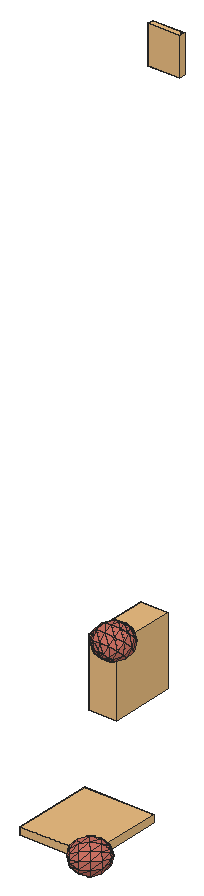
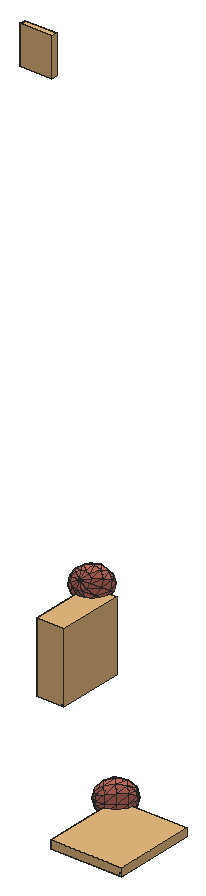
# SketchUp Ruby script. Lengths in inches.
U = 1.inch
M = Sketchup.active_model
def pt(a) = Geom::Point3d.new(a.map { |v| v * U })
def face(e, loops, mat)
  f = e.add_face(loops[0].map { |a| pt(a) })
  loops[1..].each { |l| e.add_face(l.map { |a| pt(a) }).erase! }
  f.material = f.back_material = mat if mat
  f
end
# faces: each face lists its corners as indices into pts; further lists are holes
def faces(e, pts, list, mat = nil) = list.each { |f| face(e, (f[0].is_a?(Array) ? f : [f]).map { |l| l.map { |i| pts[i] } }, mat) }
# xy, xz, yz: faces in a plane at the given z, y or x. An outline is a flat list of corners, or four numbers for a rectangle; further outlines are holes
def ring(l) = l.size == 4 ? [[l[0], l[1]], [l[2], l[1]], [l[2], l[3]], [l[0], l[3]]] : l.each_slice(2).to_a
def flat(e, list, mat, &to3) = list.each { |f| face(e, (f[0].is_a?(Array) ? f : [f]).map { |l| ring(l).map { |u, v| to3.(u, v) } }, mat) }
def xy(e, z, list, mat = nil) = flat(e, list, mat) { |x, y| [x, y, z] }
def xz(e, y, list, mat = nil) = flat(e, list, mat) { |x, z| [x, y, z] }
def yz(e, x, list, mat = nil) = flat(e, list, mat) { |y, z| [x, y, z] }
def lines(e, pts, list) = list.each { |a, b| e.add_line(pt(pts[a]), pt(pts[b])) }
# prism: a flat outline (further loops are holes) pulled along v
def prism(e, loops, v, mat = nil)
  f = face(e, loops, mat); d = Geom::Vector3d.new(v.map { |x| x * U })
  f.pushpull(f.normal.samedirection?(d) ? d.length : -d.length)
end
def box(e, o, s, mat = nil) = prism(e, [[o, [o[0] + s[0], o[1], o[2]], [o[0] + s[0], o[1] + s[1], o[2]], [o[0], o[1] + s[1], o[2]]]], [0, 0, s[2]], mat)
def at(x, y, z, deg = 0) = Geom::Transformation.translation(pt([x, y, z])) * Geom::Transformation.rotation(ORIGIN, Z_AXIS, deg.degrees)
def axes(o, x, y, z) = Geom::Transformation.new([*x, 0, *y, 0, *z, 0, *pt(o).to_a, 1])
def part(name) = M.definitions.add(name)
# library, detail: a bought-in or finely detailed component or shape, given as its bounding box
def library(name, o, s) = part(name).tap { |d| box(d.entities, o, s) }
def detail(e, o, s) = box(e.add_group.entities, o, s)
def put(e, d, t, mat = nil) = e.add_instance(d, t).tap { |i| i.material = mat if mat }
def group(e, t, mat = nil) = e.add_group.tap { |g| g.transformation = t; g.material = mat if mat }.entities
root = M.entities
M.materials.add("green").color = [174, 139, 102]
M.materials.add("vio").color = [206, 114, 100]
c1 = part("3DGeom~190_Defintion")
p = [[103.5625,-60.76,-498.22],[-159.65,90.28,-476.73],[101.5,52.12,-500],[335.44,0,-389.29],[150.07,151.03,-458.14],[-75.51,261.6,-404.23],
  [155.72,-157.36,-453.28],[-156.07,-105.24,-473.65],[-378.01,104.24,-325.73],[-280.86,302.07,-242.01],[-280.86,302.07,-242.01],[-65.73,-272.55,-395.81],
  [-373.88,-121.52,-322.17],[236.28,209.48,-383.86],[73.81,362.83,-275.57],[73.81,362.83,-275.57],[243.99,-211.79,-377.22],[-75.51,261.6,-404.23],
  [-280.86,302.07,-242.01],[-108.44,418.95,-93.44],[-75.51,261.6,-404.23],[73.81,362.83,-275.57],[87.16,-366.83,-264.07],[-269.57,-314.71,-232.28],
  [-65.73,-272.55,-395.81],[87.16,-366.83,-264.07],[-269.57,-314.71,-232.28],[344.72,-209.48,-290.42],[430.93,-151.03,-216.13],[344.72,-209.48,-290.42],
  [335.44,0,-389.29],[479.51,-52.12,-174.27],[335.44,0,-389.29],[477.44,60.76,-176.05],[335.44,0,-389.29],[337.02,211.79,-297.06],
  [425.29,157.36,-221],[335.44,0,-389.29],[337.02,211.79,-297.06],[335.44,0,-389.29],[236.28,209.48,-383.86],[248.29,366.83,-125.23],
  [236.28,209.48,-383.86],[248.29,366.83,-125.23],[337.02,211.79,-297.06],[344.72,-209.48,-290.42],[87.16,-366.83,-264.07],[243.99,-211.79,-377.22],
  [-373.88,-121.52,-322.17],[-495.09,90.28,-87.4375],[-378.01,104.24,-325.73],[-378.01,104.24,-325.73],[-410.95,261.6,-14.9375],[-378.01,104.24,-325.73],
  [-410.95,261.6,-14.9375],[-280.86,302.07,-242.01],[-269.57,-314.71,-232.28],[-491.51,-105.24,-84.36],[-373.88,-121.52,-322.17],[-373.88,-121.52,-322.17],
  [401.18,272.55,6.52],[248.29,366.83,-125.23],[344.72,-209.48,-290.42],[261.64,-362.83,-113.72],[87.16,-366.83,-264.07],[261.64,-362.83,-113.72],
  [344.72,-209.48,-290.42],[93.03,423.58,80.16],[248.29,366.83,-125.23],[87.16,-366.83,-264.07],[-93.03,-423.58,-80.16],[-269.57,-314.71,-232.28],
  [87.16,-366.83,-264.07],[-410.95,261.6,-14.9375],[-261.64,362.83,113.72],[-401.18,-272.55,-6.52],[-269.57,-314.71,-232.28],[-269.57,-314.71,-232.28],
  [-401.18,-272.55,-6.52],[491.51,105.23,84.36],[410.95,-261.6,14.9375],[261.64,-362.83,-113.72],[495.09,-90.28,87.44],[248.29,366.83,-125.23],
  [269.57,314.71,232.28],[401.18,272.55,6.52],[248.29,366.83,-125.23],[269.57,314.71,232.28],[108.44,-418.95,93.44],[410.95,-261.6,14.9375],
  [-87.16,366.83,264.07],[-479.51,52.12,174.27],[-430.93,151.03,216.13],[-410.95,261.6,-14.9375],[-477.44,-60.76,176.05],[-248.29,-366.83,125.23],
  [-401.18,-272.55,-6.52],[-410.95,261.6,-14.9375],[-344.72,209.48,290.42],[-410.95,261.6,-14.9375],[-344.72,209.48,290.42],[-261.64,362.83,113.72],
  [-248.29,-366.83,125.23],[-425.29,-157.36,221],[373.88,121.52,322.17],[269.57,314.71,232.28],[410.95,-261.6,14.9375],[280.86,-302.07,242.01],
  [280.86,-302.07,242.01],[65.73,272.55,395.81],[65.73,272.55,395.81],[269.57,314.71,232.28],[378.01,-104.24,325.73],[280.86,-302.07,242.01],
  [-73.81,-362.83,275.57],[-344.72,209.48,290.42],[-243.99,211.79,377.22],[-243.99,211.79,377.22],[-248.29,-366.83,125.23],[-337.02,-211.79,297.06],
  [-337.02,-211.79,297.06],[-335.44,0,389.29],[-344.72,209.48,290.42],[269.57,314.71,232.28],[65.73,272.55,395.81],[156.07,105.24,473.65],
  [269.57,314.71,232.28],[373.88,121.52,322.17],[75.51,-261.6,404.23],[378.01,-104.24,325.73],[75.51,-261.6,404.23],[280.86,-302.07,242.01],
  [-87.16,366.83,264.07],[-243.99,211.79,377.22],[-155.72,157.36,453.28],[-87.16,366.83,264.07],[-236.28,-209.48,383.86],[-337.02,-211.79,297.06],
  [75.51,-261.6,404.23],[-236.28,-209.48,383.86],[-73.81,-362.83,275.57],[-344.72,209.48,290.42],[-335.44,0,389.29],[-337.02,-211.79,297.06],
  [-236.28,-209.48,383.86],[-335.44,0,389.29],[373.88,121.52,322.17],[159.65,-90.28,476.73],[378.01,-104.24,325.73],[373.88,121.52,322.17],
  [378.01,-104.24,325.73],[75.51,-261.6,404.23],[-335.44,0,389.29],[75.51,-261.6,404.23],[-150.07,-151.03,458.14],[-236.28,-209.48,383.86],
  [-236.28,-209.48,383.86],[-335.44,0,389.29],[-101.5,-52.12,500],[-335.44,0,389.29],[-103.5625,60.76,498.22],[-335.44,0,389.29],
  [-335.44,0,389.29],[75.51,-261.6,404.23]]
faces(c1.entities,p,[[0,1,2],[0,2,3],[2,4,3],[2,1,5],[2,5,4],[6,7,0],[6,0,3],[0,7,1],
  [7,8,1],[1,8,9],[1,10,5],[11,12,7],[6,11,7],[7,12,8],[4,13,3],[4,5,14],
  [4,15,13],[16,11,6],[16,6,3],[17,18,19],[20,19,21],[22,23,24],[16,25,11],[11,26,12],
  [27,16,3],[28,29,30],[31,28,32],[33,31,34],[13,35,3],[36,33,37],[38,36,39],[40,21,41],
  [42,43,44],[45,46,47],[48,49,50],[51,49,52],[53,54,55],[56,57,58],[59,57,49],[38,60,36],
  [38,61,60],[62,63,64],[28,65,66],[21,19,67],[21,67,68],[69,70,71],[63,70,72],[18,73,74],
  [18,74,19],[70,75,76],[77,78,57],[36,79,33],[36,60,79],[28,80,81],[31,80,28],[33,79,82],
  [33,82,31],[31,82,80],[83,84,85],[86,67,87],[63,88,70],[89,88,63],[19,74,90],[19,90,67],
  [57,91,49],[49,91,92],[49,92,93],[78,94,57],[57,94,91],[70,95,96],[88,95,70],[97,92,98],
  [99,100,101],[102,103,78],[78,103,94],[60,104,79],[60,105,104],[106,107,88],[82,108,80],[67,90,109],
  [67,110,111],[79,104,112],[79,112,82],[82,112,113],[88,114,95],[107,114,88],[74,115,116],[74,117,90],
  [118,119,103],[114,120,95],[91,94,121],[92,91,121],[94,103,121],[122,92,121],[103,119,121],[123,124,125],
  [126,125,127],[107,128,114],[129,130,131],[132,133,134],[135,134,124],[114,136,137],[138,139,140],[133,141,142],
  [143,144,145],[146,147,148],[149,125,147],[150,147,151],[134,133,152],[153,154,155],[156,154,157],[154,158,159],
  [158,160,161],[160,134,162],[124,134,160],[124,160,125],[147,154,163],[147,158,154],[125,158,147],[125,160,158]],"vio")
c2 = part("3DGeom~191_Defintion")
p = [[58.83,-275.51,-375.83],[-159.55,-167.25,-431.01],[-6.51,0,-500],[191.37,-130.67,-435.58],[-202.64,130.67,-430.45],[148.28,167.25,-435.02],
  [-68.59,275.51,-374.17],[261.44,-309.94,-219.95],[261.44,-309.94,-219.95],[337.97,-226.32,-254.44],[337.97,-226.32,-254.44],[325.42,14.17,-379.3],
  [325.42,14.17,-379.3],[325.42,14.17,-379.3],[263.34,289.68,-253.47],[31.05,381.54,-216.95],[31.05,381.54,-216.95],[263.34,289.68,-253.47],
  [-36.6875,-381.54,-216.07],[-269.84,-289.68,-246.53],[-36.6875,-381.54,-216.07],[-335.18,-14.17,-370.7],[-344.47,226.32,-245.5625],[-267.08,309.94,-213.07],
  [-267.08,309.94,-213.07],[337.97,-226.32,-254.44],[325.42,14.17,-379.3],[415.36,-142.7,-221.95],[415.36,-142.7,-221.95],[325.42,14.17,-379.3],
  [425.06,120.2,-222.07],[325.42,14.17,-379.3],[263.34,289.68,-253.47],[425.06,120.2,-222.07],[206.3,-371.16,-127.71],[-36.6875,-381.54,-216.07],
  [58.83,-275.51,-375.83],[206.3,-371.16,-127.71],[58.83,-275.51,-375.83],[261.44,-309.94,-219.95],[-68.59,275.51,-374.17],[-267.08,309.94,-213.07],
  [-209.55,371.16,-122.29],[-68.59,275.51,-374.17],[31.05,381.54,-216.95],[-430.69,-120.2,-210.9375],[-430.69,-120.2,-210.9375],[-420.99,142.7,-211.06],
  [-335.18,-14.17,-370.7],[-420.99,142.7,-211.06],[261.44,-309.94,-219.95],[337.97,-226.32,-254.44],[394.01,-261.34,-5.125],[394.01,-261.34,-5.125],
  [263.34,289.68,-253.47],[307.83,334.49,-4.01],[263.34,289.68,-253.47],[69.59,420.35,-0.9],[263.34,289.68,-253.47],[307.83,334.49,-4.01],
  [-69.59,-420.35,0.9],[-307.83,-334.49,4.01],[-269.84,-289.68,-246.53],[-269.84,-289.68,-246.53],[-307.83,-334.49,4.01],[-430.69,-120.2,-210.9375],
  [-269.84,-289.68,-246.53],[-344.47,226.32,-245.5625],[-420.99,142.7,-211.06],[-394.01,261.34,5.125],[-267.08,309.94,-213.07],[-344.47,226.32,-245.5625],
  [472.89,-81.48,-131.17],[463.59,159.01,-6.03],[394.01,-261.34,-5.125],[206.3,-371.16,-127.71],[394.01,-261.34,-5.125],[-187.3,393.57,2.4375],
  [187.3,-393.57,-2.4375],[206.3,-371.16,-127.71],[-209.55,371.16,-122.29],[-267.08,309.94,-213.07],[-430.69,-120.2,-210.9375],[-476.14,81.48,-118.83],
  [-420.99,142.7,-211.06],[-420.99,142.7,-211.06],[-307.83,-334.49,4.01],[-463.59,-159.01,6.03],[-430.69,-120.2,-210.9375],[-430.69,-120.2,-210.9375],
  [495.13,-59.08,-6.44],[394.01,-261.34,-5.125],[206.3,-371.16,-127.71],[394.01,-261.34,-5.125],[-394.01,261.34,5.125],[-495.13,59.08,6.44],
  [476.14,-81.48,118.83],[394.01,-261.34,-5.125],[430.69,120.2,210.9375],[269.84,289.68,246.53],[269.84,289.68,246.53],[209.55,-371.16,122.29],
  [267.08,-309.94,213.07],[209.55,-371.16,122.29],[394.01,-261.34,-5.125],[344.47,-226.32,245.5625],[394.01,-261.34,-5.125],[420.99,-142.7,211.06],
  [394.01,-261.34,-5.125],[394.01,-261.34,-5.125],[307.83,334.49,-4.01],[36.6875,381.54,216.07],[269.84,289.68,246.53],[307.83,334.49,-4.01],
  [36.6875,381.54,216.07],[-206.3,371.16,127.71],[36.6875,381.54,216.07],[-31.05,-381.54,216.95],[-394.01,261.34,5.125],[-263.34,-289.68,253.47],
  [-263.34,-289.68,253.47],[-307.83,-334.49,4.01],[-472.89,81.48,131.17],[-415.36,142.7,221.95],[-337.97,226.32,254.44],[-337.97,226.32,254.44],
  [-261.44,309.94,219.95],[-261.44,309.94,219.95],[-206.3,371.16,127.71],[-263.34,-289.68,253.47],[-425.06,-120.2,222.07],[335.18,14.17,370.7],
  [335.18,14.17,370.7],[267.08,-309.94,213.07],[36.6875,381.54,216.07],[-261.44,309.94,219.95],[-325.42,-14.17,379.3],[-325.42,-14.17,379.3],
  [430.69,120.2,210.9375],[159.55,167.25,431.01],[335.18,14.17,370.7],[430.69,120.2,210.9375],[269.84,289.68,246.53],[420.99,-142.7,211.06],
  [202.64,-130.67,430.45],[344.47,-226.32,245.5625],[420.99,-142.7,211.06],[267.08,-309.94,213.07],[68.59,-275.51,374.17],[344.47,-226.32,245.5625],
  [68.59,-275.51,374.17],[267.08,-309.94,213.07],[36.6875,381.54,216.07],[-261.44,309.94,219.95],[-58.83,275.51,375.83],[36.6875,381.54,216.07],
  [-58.83,275.51,375.83],[68.59,-275.51,374.17],[-263.34,-289.68,253.47],[-31.05,-381.54,216.95],[-261.44,309.94,219.95],[-337.97,226.32,254.44],
  [-191.37,130.67,435.58],[-415.36,142.7,221.95],[-325.42,-14.17,379.3],[-415.36,142.7,221.95],[-148.28,-167.25,435.02],[-425.06,-120.2,222.07],
  [-263.34,-289.68,253.47],[-425.06,-120.2,222.07],[344.47,-226.32,245.5625],[68.59,-275.51,374.17],[68.59,-275.51,374.17],[-263.34,-289.68,253.47],
  [6.51,0,500],[68.59,-275.51,374.17]]
faces(c2.entities,p,[[0,1,2],[0,2,3],[1,4,2],[3,2,5],[2,4,6],[2,6,5],[7,0,3],[8,3,9],
  [10,3,11],[3,5,12],[13,5,14],[5,6,15],[5,16,17],[18,19,1],[20,1,0],[19,21,1],
  [1,21,4],[21,22,4],[4,22,23],[4,24,6],[25,26,27],[28,29,30],[31,32,33],[34,35,36],
  [37,38,39],[40,41,42],[43,42,44],[19,45,21],[46,47,48],[21,49,22],[50,51,52],[51,28,53],
  [30,54,55],[56,44,57],[58,57,59],[60,61,62],[60,63,35],[64,65,66],[67,68,69],[70,71,69],
  [28,30,72],[72,30,73],[30,55,73],[28,72,74],[75,50,76],[44,42,77],[44,77,57],[78,60,35],
  [78,35,79],[80,81,69],[82,83,84],[85,83,69],[86,87,88],[87,83,89],[72,90,91],[72,73,90],
  [78,92,93],[77,42,94],[87,95,83],[83,95,69],[90,96,97],[90,98,96],[90,73,98],[73,99,98],
  [73,55,100],[101,78,93],[102,103,104],[105,102,106],[107,105,108],[96,107,109],[110,111,112],[113,57,114],
  [101,60,78],[57,77,115],[57,115,116],[117,61,60],[101,117,60],[115,77,118],[117,119,61],[120,87,121],
  [95,122,69],[122,123,69],[123,124,69],[125,126,69],[127,128,69],[129,130,87],[130,95,87],[130,122,95],
  [96,131,107],[96,98,132],[133,117,101],[134,115,135],[136,122,130],[137,123,122],[138,139,140],[141,142,139],
  [143,144,145],[146,140,144],[147,148,117],[149,150,151],[152,153,154],[142,155,156],[157,158,159],[156,160,161],
  [162,163,164],[162,161,165],[166,167,168],[166,164,169],[170,144,171],[142,156,139],[172,166,173],[156,161,162],
  [140,174,144],[140,139,174],[144,166,175],[139,156,162],[174,164,166],[174,162,164],[144,174,166],[139,162,174]],"vio")
c3 = library("3DGeom~11_Defintion",[-500,-49.41,-434.02],[1000,98.82,868.04])
c4 = part("3DGeom~12_Defintion")
p = [[-473.91,-42.88,-428.57],[-493.27,-23.3125,-425.27],[-480.23,-29.84,-434.02],[-473.91,-42.88,-428.57],[-480.23,-29.84,-434.02],[-475.54,-36.36,-433.07],
  [-493.27,-23.3125,-425.27],[-486.72,-25.0625,-431.16],[-480.23,-29.84,-434.02],[-480.63,-49.41,-414.38],[-493.27,-23.3125,-425.27],[-473.91,-42.88,-428.57],
  [-480.63,-49.41,-414.38],[-473.91,-42.88,-428.57],[-475.77,-47.66,-421.73],[-493.68,-42.88,-405.63],[-493.27,-23.3125,-425.27],[-480.63,-49.41,-414.38],
  [-500,-29.84,-411.07],[-493.27,-23.3125,-425.27],[-493.68,-42.88,-405.63],[-493.27,-23.3125,-425.27],[-498.13,-25.0625,-417.92],[-493.68,-42.88,-405.63],
  [-480.63,-49.41,-414.38],[-487.1875,-47.66,-408.48],[-493.68,-42.88,-405.63],[-498.37,-36.36,-406.58],[489.39,27.6,421.47],[498.07,5.37,408.95],
  [500,12.78,407.52],[489.39,27.6,421.47],[500,12.78,407.52],[498.875,20.1875,409.65],[489.39,27.6,421.47],[493.59,-0.05,413.55],
  [498.07,5.37,408.95],[489.39,27.6,421.47],[498.875,20.1875,409.65],[494.99,25.61,414.75],[489.39,27.6,421.47],[487.78,-2.04,420.08],
  [493.59,-0.05,413.55],[489.39,27.6,421.47],[482.18,-0.05,426.79],[487.78,-2.04,420.08],[489.39,27.6,421.47],[478.3,5.37,431.9],
  [482.18,-0.05,426.79],[489.39,27.6,421.47],[477.17,12.78,434.02],[478.3,5.37,431.9],[489.39,27.6,421.47],[479.1,20.1875,432.59],
  [477.17,12.78,434.02],[489.39,27.6,421.47],[483.58,25.61,428],[479.1,20.1875,432.59]]
faces(c4.entities,p,[[0,1,2],[3,4,5],[6,7,8],[9,10,11],[12,13,14],[15,16,17],[18,19,20],[21,18,22],
  [23,24,25],[18,26,27],[28,29,30],[31,32,33],[34,35,36],[37,38,39],[40,41,42],[43,44,45],
  [46,47,48],[49,50,51],[52,53,54],[55,56,57]],"green")
c5 = library("3DGeom~13_Defintion",[-468.3,-500,-197.66],[936.6,1000,395.32])
c6 = part("3DGeom~14_Defintion")
p = [[-455.16,-492.22,-183.4],[-446.73,-497.16,-180.84],[-439.77,-500,-173.64],[-436.83,-497.09,-153.74],[-455.16,-492.22,-183.4],[-439.77,-500,-173.64],
  [-449.28,-486.4,-143.61],[-455.16,-492.22,-183.4],[-436.83,-497.09,-153.74],[-467.61,-481.53,-173.27],[-455.16,-492.22,-183.4],[-464.67,-478.62,-153.38],
  [-455.16,-492.22,-183.4],[-467.61,-481.53,-173.27],[-462.81,-486.5,-180.63],[-464.67,-478.62,-153.38],[-455.16,-492.22,-183.4],[-449.28,-486.4,-143.61],
  [-436.83,-497.09,-153.74],[-439.77,-500,-173.64],[-436.15,-499.97,-163.72],[-467.61,-481.53,-173.27],[-464.67,-478.62,-153.38],[-468.3,-478.65,-163.3],
  [-449.28,-486.4,-143.61],[-436.83,-497.09,-153.74],[-441.64,-492.12,-146.38],[-464.67,-478.62,-153.38],[-449.28,-486.4,-143.61],[-457.71,-481.46,-146.17],
  [456.2,493.0625,159.13],[456.82,479.16,194.97],[464.16,476.9375,187.85],[456.2,493.0625,159.13],[464.16,476.9375,187.85],[468.3,477.81,178.18],
  [456.2,493.0625,159.13],[468.3,477.81,178.18],[468.13,481.53,168.58],[456.2,493.0625,159.13],[448.25,483.875,197.66],[456.82,479.16,194.97],
  [456.2,493.0625,159.13],[468.13,481.53,168.58],[463.7,487.12,161.6],[456.2,493.0625,159.13],[440.74,489.82,195.18],[448.25,483.875,197.66],
  [456.2,493.0625,159.13],[436.3125,495.41,188.21],[440.74,489.82,195.18],[456.2,493.0625,159.13],[436.15,499.13,178.6],[436.3125,495.41,188.21],
  [456.2,493.0625,159.13],[440.29,500,168.94],[436.15,499.13,178.6],[456.2,493.0625,159.13],[447.63,497.78,161.8125],[440.29,500,168.94]]
faces(c6.entities,p,[[0,1,2],[3,4,5],[6,7,8],[9,10,11],[12,13,14],[15,16,17],[18,19,20],[21,22,23],
  [24,25,26],[27,28,29],[30,31,32],[33,34,35],[36,37,38],[39,40,41],[42,43,44],[45,46,47],
  [48,49,50],[51,52,53],[54,55,56],[57,58,59]],"green")
c7 = library("3DGeom~27_Defintion",[-78.21,-500,-418.56],[156.42,1000,837.12])
c8 = part("3DGeom~28_Defintion")
p = [[46.32,-458.84,-418.56],[37.22,-500,-363.86],[12.49,-468.47,-409.44],[75.6,-469.79,-400.32],[37.22,-500,-363.86],[75.6,-469.79,-400.32],
  [63.93,-461.98,-412.26],[12.49,-468.47,-409.44],[27.49,-461.21,-417.52],[12.49,-468.47,-409.44],[37.22,-500,-363.86],[7.94,-489.05,-382.09],
  [12.49,-468.47,-409.44],[7.94,-489.05,-382.09],[5.33,-478.66,-396.47],[71.06,-490.37,-372.98],[37.22,-500,-363.86],[75.6,-469.79,-400.32],
  [71.06,-490.37,-372.98],[75.6,-469.79,-400.32],[78.21,-480.18,-385.94],[37.22,-500,-363.86],[19.61,-496.86,-370.16],[7.94,-489.05,-382.09],
  [37.22,-500,-363.86],[71.06,-490.37,-372.98],[56.05,-497.625,-364.89],[-47.11,487.39,418.56],[-36.4375,500,347.21],[-55.37,499.54,349.35],
  [-47.11,487.39,418.56],[-18.93,498.77,354.62],[-36.4375,500,347.21],[-47.11,487.39,418.56],[-55.37,499.54,349.35],[-70.66,497.51,360.48],
  [-47.11,487.39,418.56],[-7.55,496.1875,369.6],[-18.93,498.77,354.62],[-47.11,487.39,418.56],[-70.66,497.51,360.48],[-78.21,494.45,377.62],
  [-47.11,487.39,418.56],[-5.33,492.93,388.15],[-7.55,496.1875,369.6],[-47.11,487.39,418.56],[-78.21,494.45,377.62],[-76,491.2,396.16],
  [-47.11,487.39,418.56],[-12.88,489.88,405.28],[-5.33,492.93,388.15],[-47.11,487.39,418.56],[-76,491.2,396.16],[-64.61,488.61,411.15],
  [-47.11,487.39,418.56],[-28.17,487.85,416.41],[-12.88,489.88,405.28]]
faces(c8.entities,p,[[0,1,2],[3,4,0],[5,0,6],[0,7,8],[9,10,11],[12,13,14],[15,16,17],[18,19,20],
  [21,22,23],[24,25,26],[27,28,29],[30,31,32],[33,34,35],[36,37,38],[39,40,41],[42,43,44],
  [45,46,47],[48,49,50],[51,52,53],[54,55,56]],"green")
g1 = group(root,at(15.3125,134.49,26.21))
put(g1,c1,axes([2.9,-0.75,9.71],[0,0.00038,0],[0,0,-0.00038],[-0.00038,0,0]),"vio")
g2 = group(root,at(15.3125,134.49,26.21))
put(g2,c2,axes([3.03,-0.6,11.73],[0,0.00039,0],[0,0,-0.00039],[-0.00039,0,0]),"vio")
g3 = group(root,at(15.3125,134.49,26.21))
put(g3,c3,axes([2.51,-0.3,9.67],[0,0.00085,0],[0,0,-0.00085],[-0.00085,0,0]),"green")
put(g3,c4,axes([2.51,-0.3,9.67],[0,0.00085,0],[0,0,-0.00085],[-0.00085,0,0]),"green")
g4 = group(root,at(15.3125,134.49,26.21))
put(g4,c5,axes([2.91,-0.25,11.34],[0,0.00073,0],[0,0,-0.00073],[-0.00073,0,0]),"green")
put(g4,c6,axes([2.91,-0.25,11.34],[0,0.00073,0],[0,0,-0.00073],[-0.00073,0,0]),"green")
g5 = group(root,at(15.3125,134.49,26.21))
put(g5,c7,axes([3.02,0.11,17.03],[0,0.0004,0],[0,0,-0.0004],[-0.0004,0,0]),"green")
put(g5,c8,axes([3.02,0.11,17.03],[0,0.0004,0],[0,0,-0.0004],[-0.0004,0,0]),"green")
